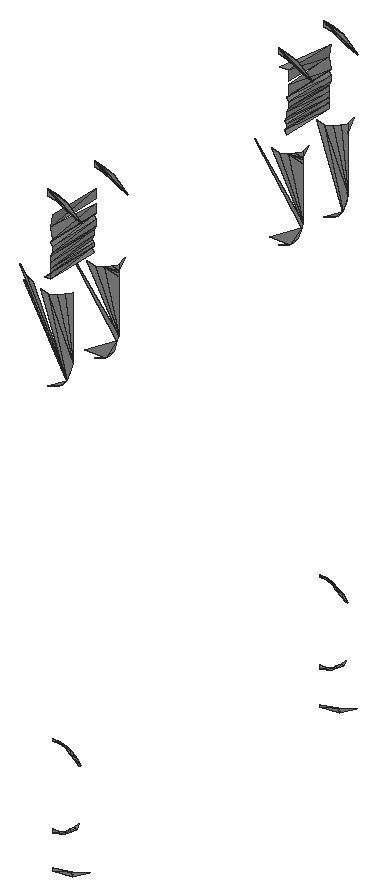
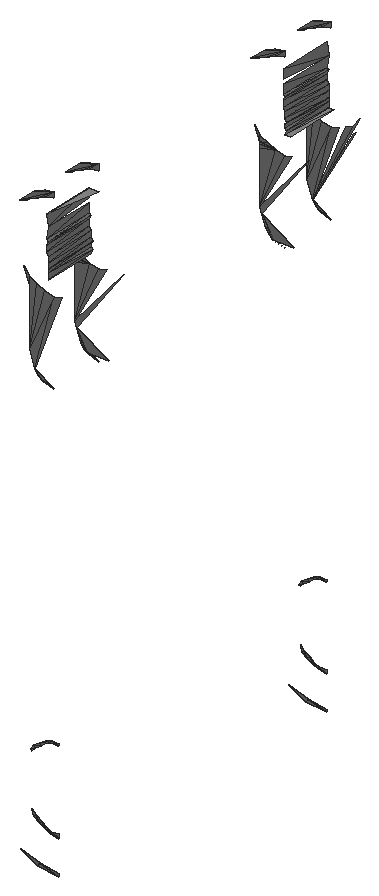
# SketchUp Ruby script. Lengths in inches.
U = 1.inch
M = Sketchup.active_model
def pt(a) = Geom::Point3d.new(a.map { |v| v * U })
def face(e, loops, mat)
  f = e.add_face(loops[0].map { |a| pt(a) })
  loops[1..].each { |l| e.add_face(l.map { |a| pt(a) }).erase! }
  f.material = f.back_material = mat if mat
  f
end
# faces: each face lists its corners as indices into pts; further lists are holes
def faces(e, pts, list, mat = nil) = list.each { |f| face(e, (f[0].is_a?(Array) ? f : [f]).map { |l| l.map { |i| pts[i] } }, mat) }
# xy, xz, yz: faces in a plane at the given z, y or x. An outline is a flat list of corners, or four numbers for a rectangle; further outlines are holes
def ring(l) = l.size == 4 ? [[l[0], l[1]], [l[2], l[1]], [l[2], l[3]], [l[0], l[3]]] : l.each_slice(2).to_a
def flat(e, list, mat, &to3) = list.each { |f| face(e, (f[0].is_a?(Array) ? f : [f]).map { |l| ring(l).map { |u, v| to3.(u, v) } }, mat) }
def xy(e, z, list, mat = nil) = flat(e, list, mat) { |x, y| [x, y, z] }
def xz(e, y, list, mat = nil) = flat(e, list, mat) { |x, z| [x, y, z] }
def yz(e, x, list, mat = nil) = flat(e, list, mat) { |y, z| [x, y, z] }
def lines(e, pts, list) = list.each { |a, b| e.add_line(pt(pts[a]), pt(pts[b])) }
# prism: a flat outline (further loops are holes) pulled along v
def prism(e, loops, v, mat = nil)
  f = face(e, loops, mat); d = Geom::Vector3d.new(v.map { |x| x * U })
  f.pushpull(f.normal.samedirection?(d) ? d.length : -d.length)
end
def box(e, o, s, mat = nil) = prism(e, [[o, [o[0] + s[0], o[1], o[2]], [o[0] + s[0], o[1] + s[1], o[2]], [o[0], o[1] + s[1], o[2]]]], [0, 0, s[2]], mat)
def at(x, y, z, deg = 0) = Geom::Transformation.translation(pt([x, y, z])) * Geom::Transformation.rotation(ORIGIN, Z_AXIS, deg.degrees)
def axes(o, x, y, z) = Geom::Transformation.new([*x, 0, *y, 0, *z, 0, *pt(o).to_a, 1])
def part(name) = M.definitions.add(name)
# library, detail: a bought-in or finely detailed component or shape, given as its bounding box
def library(name, o, s) = part(name).tap { |d| box(d.entities, o, s) }
def detail(e, o, s) = box(e.add_group.entities, o, s)
def put(e, d, t, mat = nil) = e.add_instance(d, t).tap { |i| i.material = mat if mat }
def group(e, t, mat = nil) = e.add_group.tap { |g| g.transformation = t; g.material = mat if mat }.entities
root = M.entities
M.materials.add("Material \#1").color = [140, 140, 140]
xy(root,193.6091,[[101.3835,115.8116,101.3835,116.0971,101.412,116.0971],[101.3835,115.8116,101.412,116.0971,101.412,115.8116]],"Material \#1")
xy(root,193.9189,[[101.3693,117.386,101.4167,117.386,101.4167,117.6715]],"Material \#1")
xz(root,115.8208,[[101.3928,193.094,101.4476,193.109,101.4213,193.0979],[101.3928,193.094,101.4901,193.1492,101.4476,193.109],[101.4476,193.109,101.4901,193.1492,101.4707,193.1264],[101.4901,193.1492,101.2392,193.6187,101.2697,193.5827],[101.4901,193.1492,101.2654,193.54,101.2633,193.5452],
  [101.4901,193.1492,101.2669,193.5345,101.2654,193.54],[101.4901,193.1492,101.2678,193.5287,101.2669,193.5345],[101.4901,193.1492,101.2697,193.5827,101.3062,193.5553],[101.4901,193.1492,101.3477,193.5378,101.3928,193.5316],[101.4901,193.1492,101.3928,193.5316,101.5175,193.2412],
  [101.4901,193.1492,101.5142,193.2075,101.5048,193.1765],[101.4901,193.1492,101.5175,193.2412,101.5142,193.2075],[101.5175,193.2412,101.3928,193.5316,101.4379,193.5378],[101.5175,193.2412,101.4379,193.5378,101.4793,193.5553],[101.5175,193.2412,101.4793,193.5553,101.5159,193.5827],
  [101.5175,193.2412,101.5159,193.5827,101.5175,193.5227],[101.5175,193.5227,101.5187,193.5351,101.5178,193.5291],[101.5187,193.5351,101.5225,193.5456,101.5203,193.5405],[101.5668,193.9286,101.3928,194.0273,101.4909,194.0005],[101.5668,193.9286,101.4793,193.9727,101.3928,194.0273],
  [101.5668,193.9286,101.5159,193.9453,101.4793,193.9727],[101.4793,193.9727,101.4379,193.9902,101.3928,194.0273],[101.4379,193.9902,101.3928,193.9963,101.3928,194.0273],[101.4909,194.0005,101.3928,194.0273,101.4439,194.0204]],"Material \#1")
xz(root,115.8515,[[101.3928,190.7631,101.3928,190.7747,101.4942,190.7855],[101.3928,190.7631,101.4942,190.7855,101.496,190.774],[101.496,190.774,101.4942,190.7855,101.5895,190.8164],[101.3928,190.9443,101.3928,190.9559,101.4251,190.9594],[101.3928,190.9443,101.4251,190.9594,101.4269,190.9479],
  [101.4269,190.9479,101.4251,190.9594,101.4558,190.9693],[101.4269,190.9479,101.4558,190.9693,101.4592,190.9584],[101.4592,190.9584,101.4558,190.9693,101.484,190.9851],[101.4592,190.9584,101.484,190.9851,101.489,190.9751],[101.489,190.9751,101.484,190.9851,101.5092,191.0062],
  [101.489,190.9751,101.5092,191.0062,101.5156,190.9973],[101.5156,190.9973,101.5092,191.0062,101.531,191.0319],[101.531,191.3068,101.5092,191.3324,101.5385,191.3143],[101.5385,191.3143,101.5092,191.3324,101.5156,191.3414],[101.5092,191.3324,101.484,191.3535,101.5156,191.3414],
  [101.5156,191.3414,101.484,191.3535,101.489,191.3635],[101.484,191.3535,101.4558,191.3693,101.489,191.3635],[101.489,191.3635,101.4558,191.3693,101.4592,191.3802],[101.4558,191.3693,101.4251,191.3793,101.4592,191.3802],[101.4251,191.3793,101.3928,191.3827,101.4269,191.3907],
  [101.4251,191.3793,101.4269,191.3907,101.4592,191.3802],[101.3928,191.3827,101.3928,191.3944,101.4269,191.3907]],"Material \#1")
xz(root,116.1277,[[101.3928,193.094,101.4213,193.0979,101.4476,193.109],[101.338,193.109,101.4476,193.109,101.5142,193.2075],[101.4476,193.109,101.4707,193.1264,101.4901,193.1492],[101.4476,193.109,101.4901,193.1492,101.5142,193.2075],[101.4901,193.1492,101.5048,193.1765,101.5142,193.2075],
  [101.5142,193.2075,101.5175,193.2412,101.2633,193.5452],[101.5175,193.2412,101.3928,193.5316,101.3477,193.5378],[101.5175,193.2412,101.4379,193.5378,101.3928,193.5316],[101.5175,193.2412,101.5175,193.5227,101.4379,193.5378],[101.5175,193.5227,101.5187,193.5351,101.4379,193.5378],
  [101.5175,193.5227,101.5178,193.5291,101.5187,193.5351],[101.5187,193.5351,101.5225,193.5456,101.4379,193.5378],[101.5187,193.5351,101.5203,193.5405,101.5225,193.5456],[101.4379,193.5378,101.5225,193.5456,101.4793,193.5553],[101.5225,193.5456,101.5159,193.5827,101.4793,193.5553],
  [101.5225,193.5456,101.5464,193.6187,101.5159,193.5827],[101.5668,193.9286,101.3928,194.0273,101.4793,193.9727],[101.5668,193.9286,101.4909,194.0005,101.3928,194.0273],[101.5668,193.9286,101.4793,193.9727,101.5159,193.9453],[101.4793,193.9727,101.3928,194.0273,101.4379,193.9902],
  [101.4379,193.9902,101.3928,194.0273,101.3928,193.9964],[101.4909,194.0005,101.4439,194.0204,101.3928,194.0273]],"Material \#1")
xz(root,117.3553,[[101.3928,193.094,101.4476,193.109,101.4213,193.0979],[101.338,193.109,101.5142,193.2075,101.4476,193.109],[101.4476,193.109,101.49,193.1492,101.4707,193.1264],[101.4476,193.109,101.5142,193.2075,101.49,193.1492],[101.49,193.1492,101.5142,193.2075,101.5048,193.1765],
  [101.5142,193.2075,101.2633,193.5452,101.5175,193.2412],[101.5175,193.2412,101.3477,193.5378,101.3928,193.5316],[101.5175,193.2412,101.3928,193.5316,101.4379,193.5378],[101.5175,193.2412,101.4379,193.5378,101.5175,193.5227],[101.5175,193.5227,101.4379,193.5378,101.5187,193.5351],
  [101.5175,193.5227,101.5187,193.5351,101.5178,193.5291],[101.5187,193.5351,101.4379,193.5378,101.5225,193.5456],[101.5187,193.5351,101.5225,193.5456,101.5203,193.5405],[101.4379,193.5378,101.4793,193.5553,101.5225,193.5456],[101.5225,193.5456,101.4793,193.5553,101.5159,193.5827],
  [101.5225,193.5456,101.5159,193.5827,101.5464,193.6187],[101.5668,193.9286,101.3928,194.0273,101.4908,194.0005],[101.5668,193.9286,101.4793,193.9727,101.3928,194.0273],[101.5668,193.9286,101.5159,193.9453,101.4793,193.9727],[101.4793,193.9727,101.4379,193.9902,101.3928,194.0273],
  [101.4379,193.9902,101.3928,193.9964,101.3928,194.0273],[101.4908,194.0005,101.3928,194.0273,101.4439,194.0204]],"Material \#1")
xz(root,117.6316,[[101.3928,190.7631,101.4942,190.7855,101.3928,190.7747],[101.3928,190.7631,101.496,190.774,101.4942,190.7855],[101.496,190.774,101.5895,190.8164,101.4942,190.7855],[101.3928,190.9443,101.4251,190.9594,101.3928,190.9559],[101.3928,190.9443,101.4269,190.9479,101.4251,190.9594],
  [101.4269,190.9479,101.4558,190.9693,101.4251,190.9594],[101.4269,190.9479,101.4592,190.9584,101.4558,190.9693],[101.4592,190.9584,101.484,190.9851,101.4558,190.9693],[101.4592,190.9584,101.489,190.9751,101.484,190.9851],[101.489,190.9751,101.5092,191.0062,101.484,190.9851],
  [101.489,190.9751,101.5156,190.9973,101.5092,191.0062],[101.5156,190.9973,101.531,191.0319,101.5092,191.0062],[101.531,191.3068,101.5385,191.3143,101.5092,191.3324],[101.5385,191.3143,101.5156,191.3414,101.5092,191.3324],[101.5092,191.3324,101.5156,191.3414,101.484,191.3535],
  [101.5156,191.3414,101.489,191.3635,101.484,191.3535],[101.484,191.3535,101.489,191.3635,101.4558,191.3693],[101.489,191.3635,101.4592,191.3802,101.4558,191.3693],[101.4558,191.3693,101.4592,191.3802,101.4251,191.3793],[101.4251,191.3793,101.4269,191.3908,101.3928,191.3827],
  [101.4251,191.3793,101.4592,191.3802,101.4269,191.3908],[101.3928,191.3827,101.4269,191.3908,101.3928,191.3944]],"Material \#1")
xz(root,117.6622,[[101.3928,193.094,101.4213,193.0979,101.4476,193.109],[101.3928,193.094,101.4476,193.109,101.4901,193.1492],[101.4476,193.109,101.4707,193.1264,101.4901,193.1492],[101.4901,193.1492,101.3928,193.5316,101.3477,193.5378],[101.4901,193.1492,101.5175,193.2412,101.3928,193.5316],
  [101.4901,193.1492,101.5048,193.1765,101.5142,193.2075],[101.4901,193.1492,101.5142,193.2075,101.5175,193.2412],[101.5175,193.2412,101.4379,193.5378,101.3928,193.5316],[101.5175,193.2412,101.4793,193.5553,101.4379,193.5378],[101.5175,193.2412,101.5159,193.5827,101.4793,193.5553],
  [101.5175,193.2412,101.5175,193.5227,101.5159,193.5827],[101.5175,193.5227,101.5187,193.5351,101.5159,193.5827],[101.5175,193.5227,101.5178,193.5291,101.5187,193.5351],[101.5187,193.5351,101.5464,193.6187,101.5159,193.5827],[101.5187,193.5351,101.5203,193.5405,101.5225,193.5456],
  [101.5668,193.9286,101.3928,194.0273,101.4793,193.9727],[101.5668,193.9286,101.4909,194.0005,101.3928,194.0273],[101.5668,193.9286,101.4793,193.9727,101.5159,193.9453],[101.4793,193.9727,101.3928,194.0273,101.4379,193.9902],[101.4379,193.9902,101.3928,194.0273,101.3928,193.9964],
  [101.4909,194.0005,101.4439,194.0204,101.3928,194.0273]],"Material \#1")
yz(root,101.412,[[115.8116,193.6943,116.0971,193.6943,116.0971,193.7214],[115.8116,193.6943,116.0971,193.7214,115.8116,193.7214],[117.386,193.6943,117.6715,193.6943,117.386,193.7214],[117.6715,193.6943,117.6715,193.7214,117.386,193.7214]],"Material \#1")
yz(root,101.4167,[[115.8116,193.8027,116.0971,193.8027,116.0971,193.8531],[117.386,193.8027,117.6715,193.8027,117.386,193.8531]],"Material \#1")
yz(root,101.4192,[[115.8116,193.7433,116.0971,193.7433,116.0971,193.7653],[115.8116,193.7433,116.0971,193.7653,115.8116,193.7653],[117.386,193.7433,117.6715,193.7433,117.386,193.7653],[117.6715,193.7433,117.6715,193.7653,117.386,193.7653]],"Material \#1")
p = [[101.405,115.8116,193.6362],[101.4025,116.0971,193.6323],[101.4075,116.0971,193.6401],[101.405,115.8116,193.6362],[101.4075,116.0971,193.6401],[101.4075,116.0971,193.6575],
  [101.405,115.8116,193.6614],[101.4025,116.0971,193.6323],[101.405,115.8116,193.6362],[101.412,115.8116,193.6091],[101.412,115.8116,193.6091],[101.412,116.0971,193.6091],
  [101.4025,116.0971,193.6323],[101.405,117.6715,193.6362],[101.4075,117.386,193.6401],[101.4025,117.386,193.6323],[101.405,117.6715,193.6362],[101.405,117.6715,193.6614],
  [101.4075,117.386,193.6575],[101.4075,117.386,193.6401],[101.412,117.6715,193.6091],[101.405,117.6715,193.6362],[101.4025,117.386,193.6323],[101.4025,117.386,193.6323],
  [101.412,117.386,193.6091],[101.412,117.6715,193.6091],[101.405,115.8116,193.6614],[101.4075,116.0971,193.6575],[101.4025,116.0971,193.6652],[101.405,115.8116,193.6614],
  [101.4025,116.0971,193.6652],[101.412,116.0971,193.6943],[101.412,116.0971,193.6943],[101.412,115.8116,193.6943],[101.405,115.8116,193.6614],[101.412,115.8116,193.7214],
  [101.412,116.0971,193.7214],[101.4192,116.0971,193.7433],[101.4192,116.0971,193.7433],[101.4192,115.8116,193.7433],[101.412,115.8116,193.7214],[101.405,117.6715,193.6614],
  [101.4025,117.386,193.6652],[101.4075,117.386,193.6575],[101.412,117.386,193.6943],[101.4025,117.386,193.6652],[101.405,117.6715,193.6614],[101.405,117.6715,193.6614],
  [101.412,117.6715,193.6943],[101.412,117.386,193.6943],[101.412,117.6715,193.7214],[101.4192,117.6715,193.7433],[101.4192,117.386,193.7433],[101.412,117.386,193.7214],
  [101.412,115.8116,193.7872],[101.412,116.0971,193.7872],[101.4167,116.0971,193.8027],[101.412,116.0971,193.7872],[101.412,115.8116,193.7872],[101.4192,115.8116,193.7653],
  [101.4167,116.0971,193.8027],[101.4167,115.8116,193.8027],[101.412,115.8116,193.7872],[101.4167,116.0971,193.8531],[101.4142,115.8116,193.8625],[101.4167,115.8116,193.8027],
  [101.4192,115.8116,193.7653],[101.4192,116.0971,193.7653],[101.412,116.0971,193.7872],[101.4167,117.386,193.8027],[101.412,117.386,193.7872],[101.412,117.6715,193.7872],
  [101.4192,117.6715,193.7653],[101.412,117.6715,193.7872],[101.412,117.386,193.7872],[101.412,117.6715,193.7872],[101.4167,117.6715,193.8027],[101.4167,117.386,193.8027],
  [101.4167,117.6715,193.8027],[101.4142,117.6715,193.8625],[101.4167,117.386,193.8531],[101.412,117.386,193.7872],[101.4192,117.386,193.7653],[101.4192,117.6715,193.7653],
  [101.4142,115.8116,193.8625],[101.4167,116.0971,193.8685],[101.4167,116.0971,193.9189],[101.4167,116.0971,193.9189],[101.4167,115.8116,193.9189],[101.4142,115.8116,193.8625],
  [101.4167,117.386,193.9189],[101.4167,117.386,193.8685],[101.4142,117.6715,193.8625],[101.4142,117.6715,193.8625],[101.4167,117.6715,193.9189],[101.4167,117.386,193.9189]]
faces(root,p,[[0,1,2],[3,4,5],[5,6,3],[7,8,9],[10,11,12],[13,14,15],[16,17,18],[18,19,16],
  [20,21,22],[23,24,25],[26,27,28],[29,30,31],[32,33,34],[35,36,37],[38,39,40],[41,42,43],
  [44,45,46],[47,48,49],[50,51,52],[52,53,50],[54,55,56],[57,58,59],[60,61,62],[63,64,65],
  [66,67,68],[69,70,71],[72,73,74],[75,76,77],[78,79,80],[81,82,83],[84,85,86],[87,88,89],
  [90,91,92],[93,94,95]],"Material \#1")
